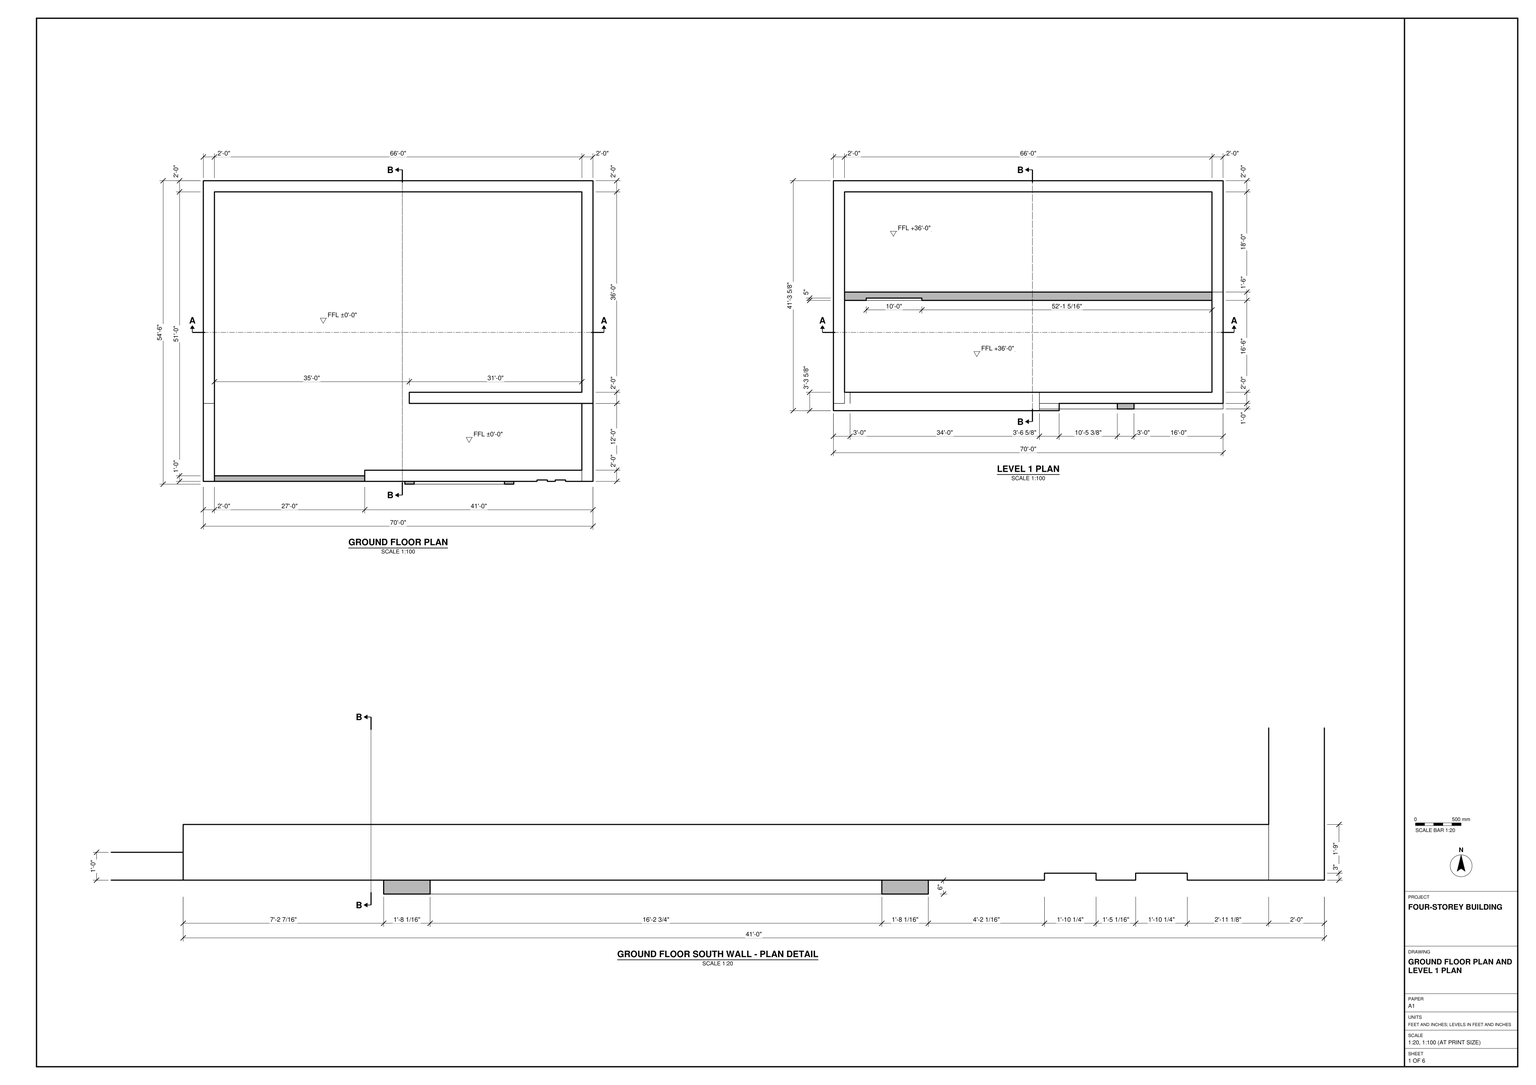
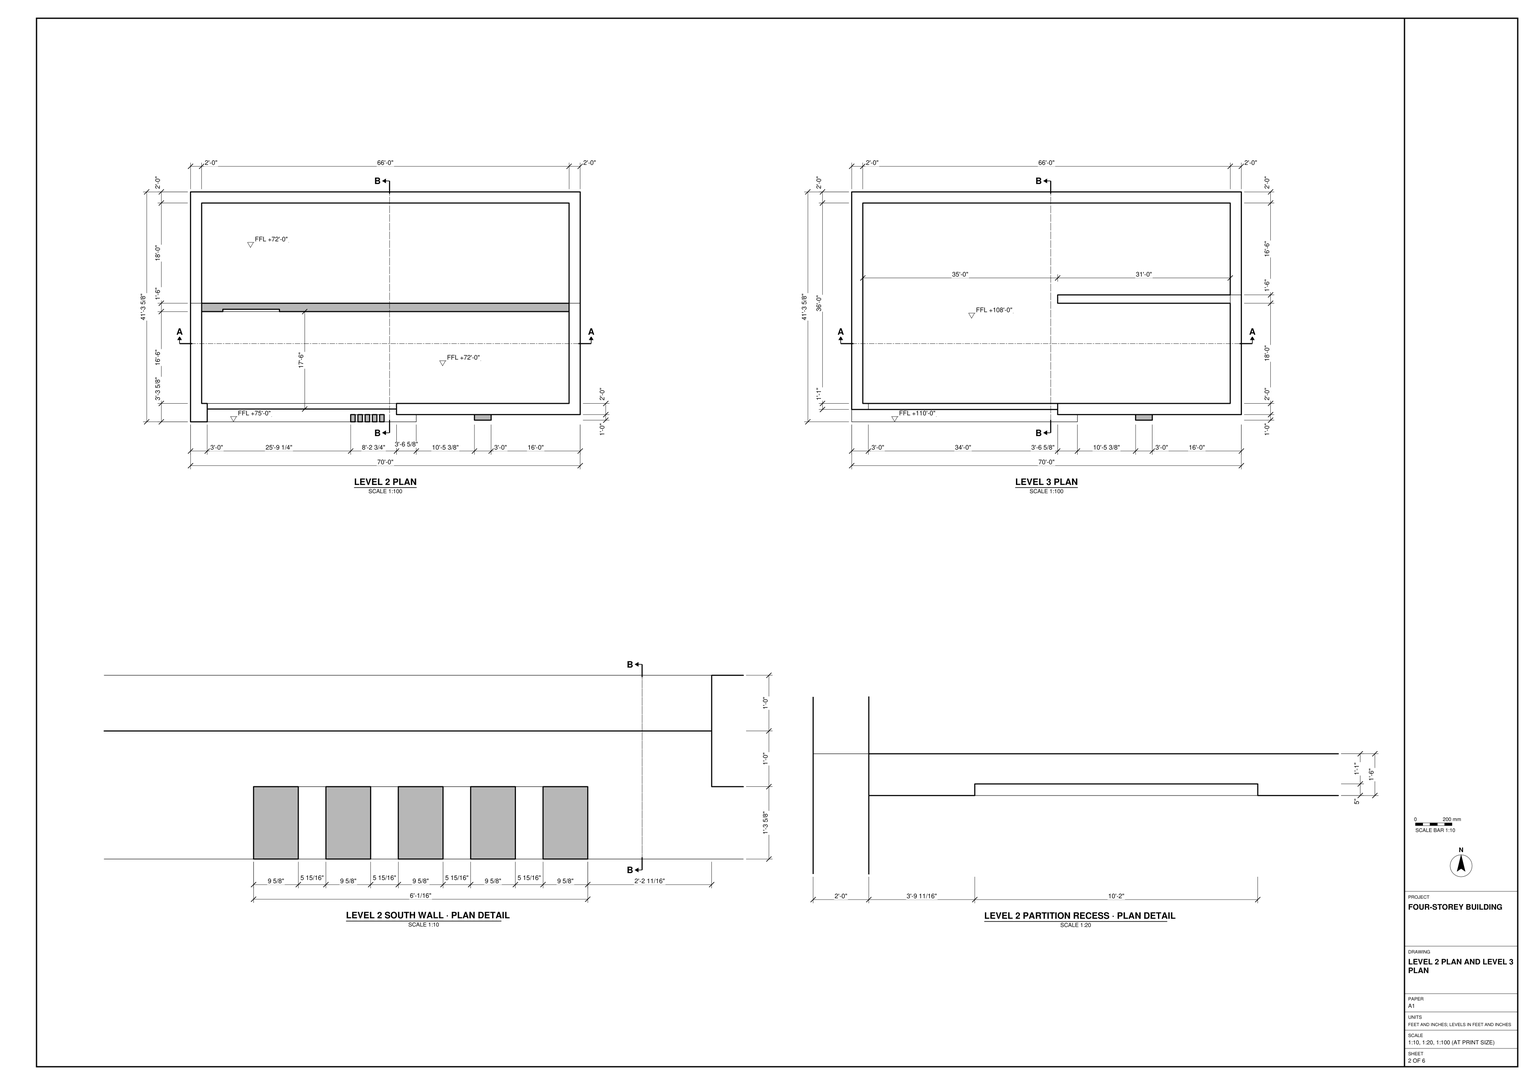
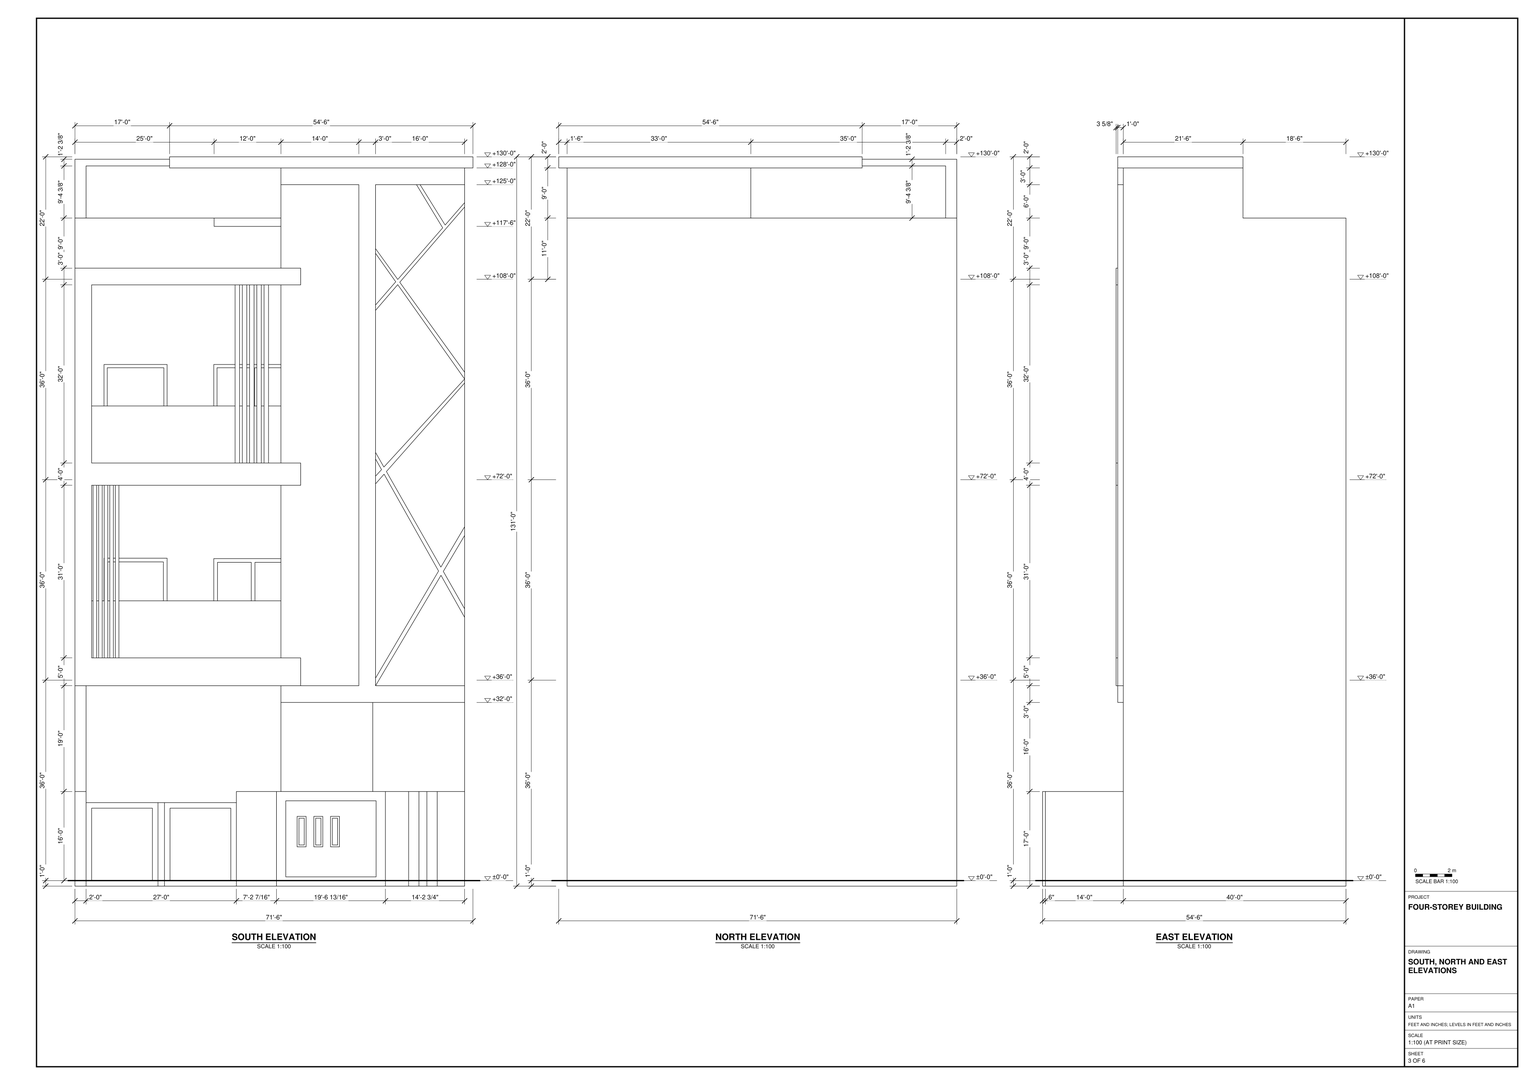
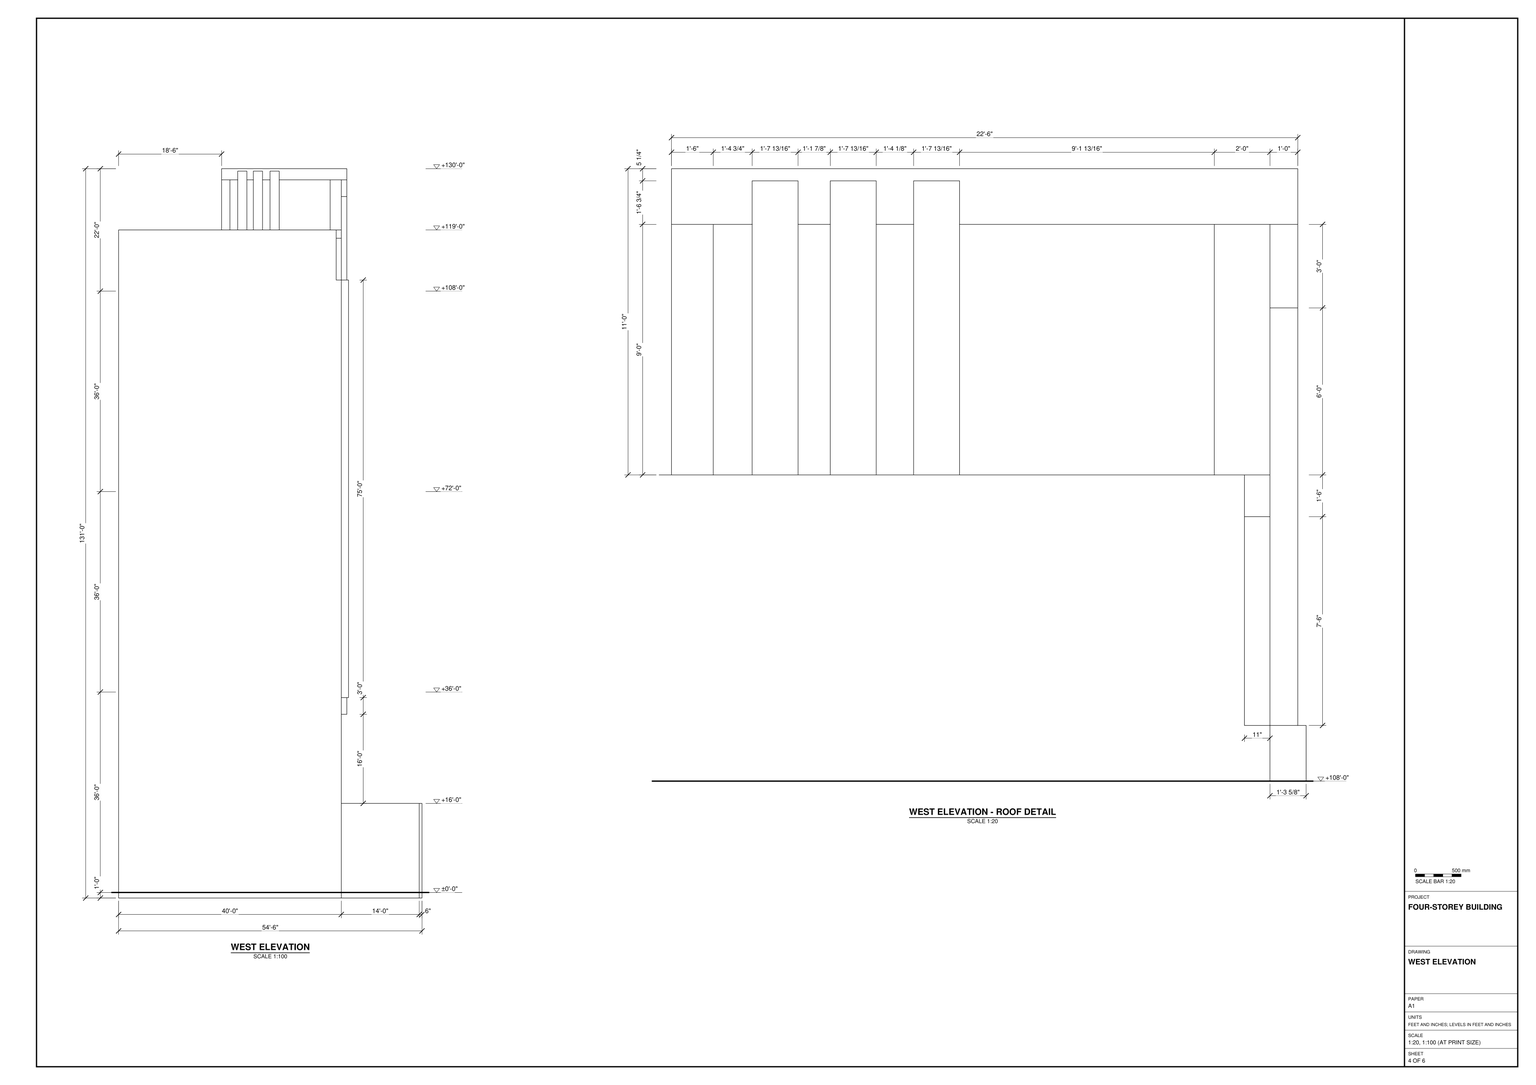
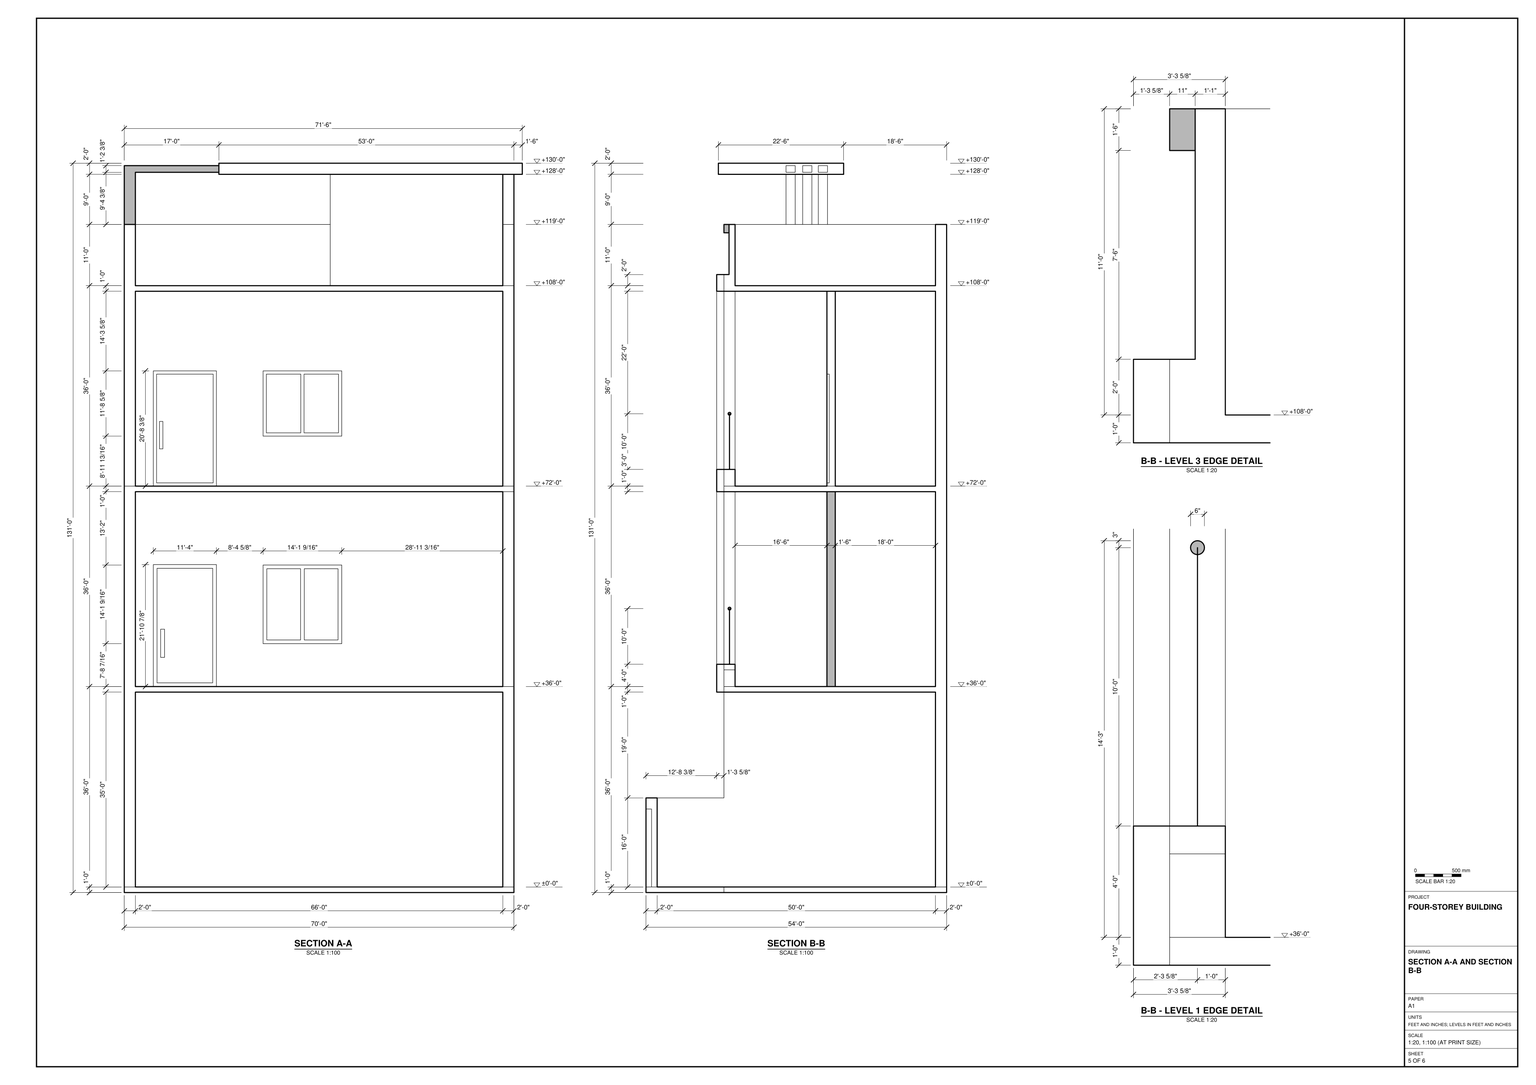
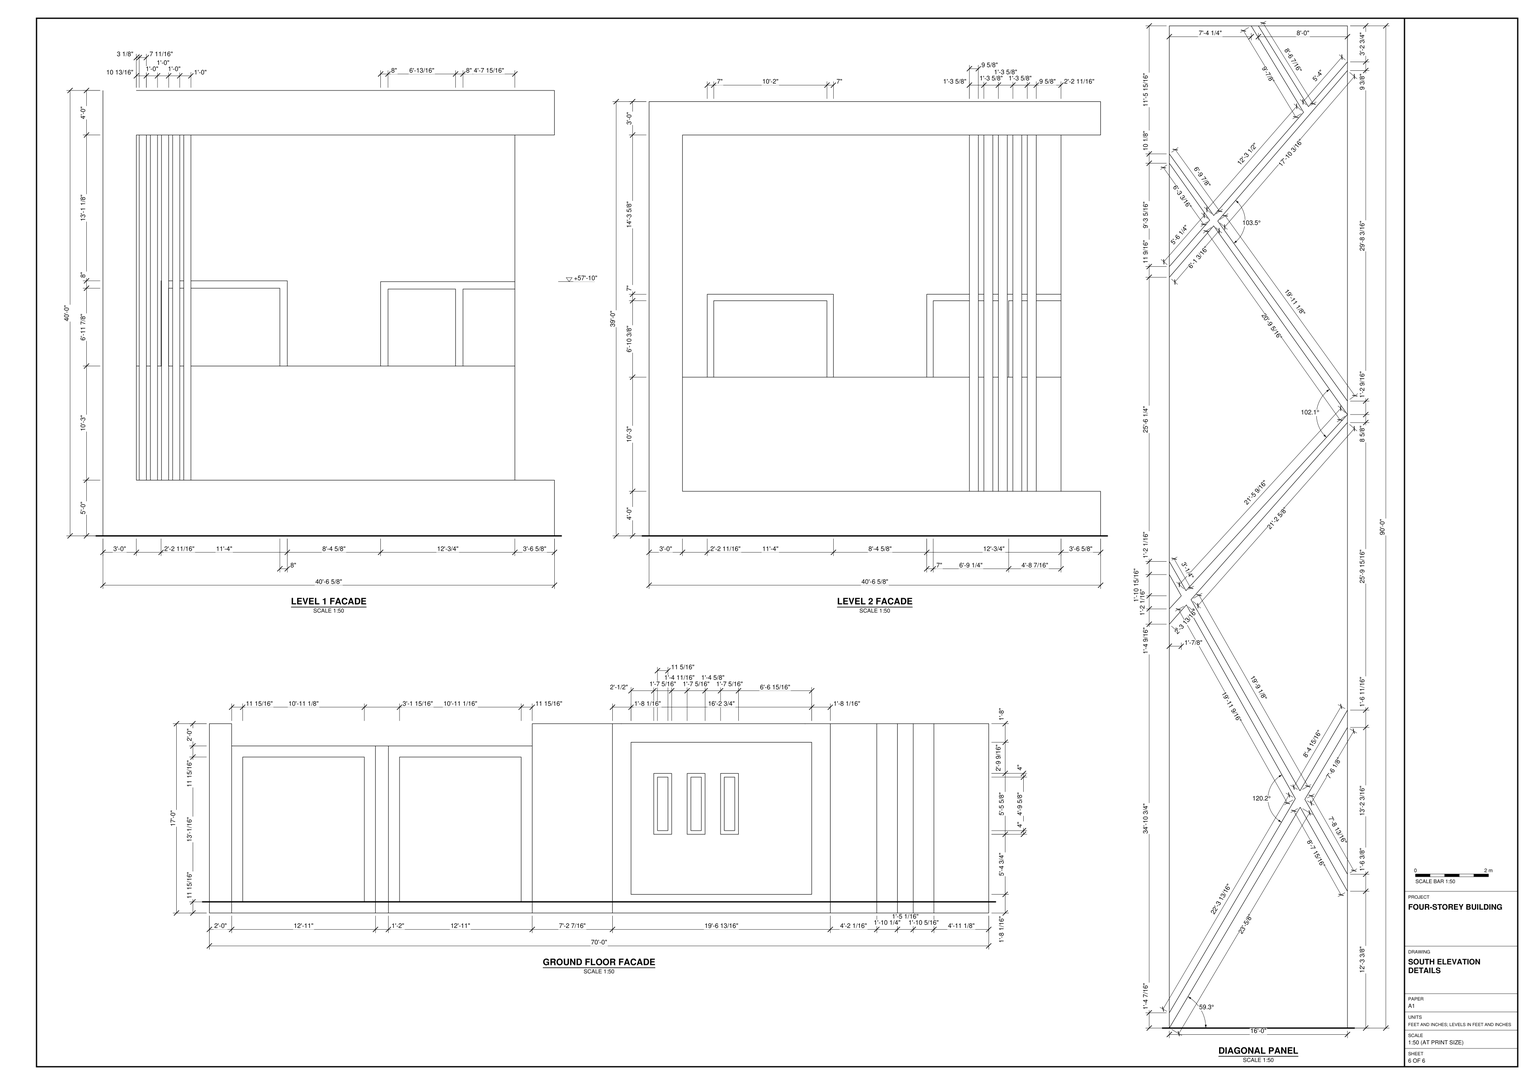
Build the four-storey building in SketchUp from task_files/diagram_01.pdf. Work in feet and inches. The overall model extents, including projections, are 71'-6" east to west, 54'-6" north to south and 131'-0" from bottom to top. Set the floor levels at ±0'-0", +36'-0", +72'-0" and +108'-0".

Use the floor plans to lay out the perimeter walls, internal partitions and slabs at their drawn thicknesses. Extend the low ground-floor frontage south of the upper-storey walls. Follow the plan details for the partition recesses and the changes in depth along the south face. On that face, model the ground-floor openings and inset panel, then form the stacked recessed bays above. Place the projecting horizontal bands and vertical fins as shown, noting that the fins change position between bays. Model the tall panel with crossing diagonal strips to the east of the bays. Use the elevations to shape the stepped roofline and its cap.

Keep walls, slabs and roof elements in separate groups or components, and keep each furniture or joinery piece shown separate. Use components for repeated parts such as the fins. Any decor or loose items shown may be represented by suitable library components. Save one SketchUp model as output_files/four_storey_building_with_its_screened_south_elevation.skp.

# SketchUp Ruby script. Lengths in inches.
U = 1.inch
M = Sketchup.active_model
def pt(a) = Geom::Point3d.new(a.map { |v| v * U })
def face(e, loops, mat)
  f = e.add_face(loops[0].map { |a| pt(a) })
  loops[1..].each { |l| e.add_face(l.map { |a| pt(a) }).erase! }
  f.material = f.back_material = mat if mat
  f
end
# faces: each face lists its corners as indices into pts; further lists are holes
def faces(e, pts, list, mat = nil) = list.each { |f| face(e, (f[0].is_a?(Array) ? f : [f]).map { |l| l.map { |i| pts[i] } }, mat) }
# xy, xz, yz: faces in a plane at the given z, y or x. An outline is a flat list of corners, or four numbers for a rectangle; further outlines are holes
def ring(l) = l.size == 4 ? [[l[0], l[1]], [l[2], l[1]], [l[2], l[3]], [l[0], l[3]]] : l.each_slice(2).to_a
def flat(e, list, mat, &to3) = list.each { |f| face(e, (f[0].is_a?(Array) ? f : [f]).map { |l| ring(l).map { |u, v| to3.(u, v) } }, mat) }
def xy(e, z, list, mat = nil) = flat(e, list, mat) { |x, y| [x, y, z] }
def xz(e, y, list, mat = nil) = flat(e, list, mat) { |x, z| [x, y, z] }
def yz(e, x, list, mat = nil) = flat(e, list, mat) { |y, z| [x, y, z] }
def lines(e, pts, list) = list.each { |a, b| e.add_line(pt(pts[a]), pt(pts[b])) }
# prism: a flat outline (further loops are holes) pulled along v
def prism(e, loops, v, mat = nil)
  f = face(e, loops, mat); d = Geom::Vector3d.new(v.map { |x| x * U })
  f.pushpull(f.normal.samedirection?(d) ? d.length : -d.length)
end
def box(e, o, s, mat = nil) = prism(e, [[o, [o[0] + s[0], o[1], o[2]], [o[0] + s[0], o[1] + s[1], o[2]], [o[0], o[1] + s[1], o[2]]]], [0, 0, s[2]], mat)
def at(x, y, z, deg = 0) = Geom::Transformation.translation(pt([x, y, z])) * Geom::Transformation.rotation(ORIGIN, Z_AXIS, deg.degrees)
def axes(o, x, y, z) = Geom::Transformation.new([*x, 0, *y, 0, *z, 0, *pt(o).to_a, 1])
def part(name) = M.definitions.add(name)
# library, detail: a bought-in or finely detailed component or shape, given as its bounding box
def library(name, o, s) = part(name).tap { |d| box(d.entities, o, s) }
def detail(e, o, s) = box(e.add_group.entities, o, s)
def put(e, d, t, mat = nil) = e.add_instance(d, t).tap { |i| i.material = mat if mat }
def group(e, t, mat = nil) = e.add_group.tap { |g| g.transformation = t; g.material = mat if mat }.entities
root = M.entities
M.materials.add("[0012_Bisque]").color = [214, 191, 164]
M.materials.add("[0012_Bisque]1").color = [255, 228, 196]
M.materials.add("[0021_DarkRed]").color = [94, 0, 0]
M.materials.add("[0021_DarkRed]1").color = [107, 0, 0]
M.materials.add("[0022_Maroon]").color = [63, 0, 0]
M.materials.add("[0027_PeachPuff]").color = [226, 194, 164]
M.materials.add("[0030_OldLace]").color = [237, 229, 215]
M.materials.add("[0042_Sienna]").color = [117, 60, 32]
M.materials.add("[0048_PaleGoldenrod]").color = [238, 232, 170]
M.materials.add("[0136_Charcoal]").color = [35, 35, 35]
M.materials.add("[Cladding Siding Tan]").color = [204, 97, 36]
M.materials.add("[Cladding Stucco White]").color = [200, 200, 200]
M.materials.add("[Granite Brown]").color = [126, 104, 91]
M.materials.add("[Granite Dark Gray]").color = [69, 68, 68]
M.materials.add("[Modern Siding]").color = [191, 132, 100]
M.materials.add("[Stone Flagstone Ashlar]").color = [175, 116, 102]
M.materials.add("[Stone Masonry Multi]").color = [182, 175, 164]
M.materials.add("[Translucent Glass Gray]").color = [198, 198, 198]
M.materials["[Translucent Glass Gray]"].alpha = 0.5
M.materials.add("[Translucent Glass Gray]1").color = [128, 128, 128]
M.materials["[Translucent Glass Gray]1"].alpha = 0.5
M.materials.add("[Wood Bamboo]").color = [177, 105, 43]
M.materials.add("[Wood Cherry Original]").color = [152, 86, 42]
xy(root,0,[[0,6,24,174],[24,6,24,174,840,174,840,6,780.9,6,780.9,9,758.64,9,758.64,6,741.58,6,741.58,9,719.33,9,719.33,6],[0,174,840,654]])
xy(root,0,[[434.43,0,669.25,6]],"[0012_Bisque]1")
xy(root,12,[[24,18,348,18,348,30,816,30,816,174,444,174,444,198,816,198,816,630,24,630]],"[Granite Dark Gray]")
xy(root,20.04,[[454.47,0,649.21,6]],"[0012_Bisque]1")
xy(root,84.76,[[478.96,0,498.27,6],[514.96,0,534.27,6],[550.96,0,570.27,6]])
xy(root,88.76,[[482.96,0,494.27,6],[518.96,0,530.27,6],[554.96,0,566.27,6]])
xy(root,146.39,[[482.96,0,494.27,6],[518.96,0,530.27,6],[554.96,0,566.27,6]])
xy(root,150.39,[[478.96,0,498.27,6],[514.96,0,534.27,6],[550.96,0,570.27,6]])
xy(root,180,[[24,6,348,18]])
xy(root,183.96,[[454.47,0,649.21,6]],"[0012_Bisque]1")
xy(root,204,[[0,6,24,174]],"[0012_Bisque]")
xy(root,204,[[434.43,0,669.25,6],[348,6,719.33,6,719.33,9,741.58,9,741.58,6,758.64,6,758.64,9,780.9,9,780.9,6,840,6,840,174,816,174,816,30,348,30]],"[0012_Bisque]1")
xy(root,396,[[444,162,840,174]],"[0012_Bisque]1")
xy(root,432,[[444,158.4,486.63,162],[444,162,486.63,174]])
xy(root,432,[[486.63,162,612,174],[648,162,840,174]],"[0012_Bisque]1")
xy(root,432,[[0,158.4,0,174,24,174,24,630,816,630,816,198,444,198,444,158.4]],"[Wood Cherry Original]")
xy(root,444,[[24,396,816,414],[24,414,816,630]])
xy(root,444,[[24,198,816,396]],"[Granite Brown]")
xy(root,452,[[70.68,396,190.68,401]],"[0022_Maroon]")
xy(root,492,[[36,158.4,39.12,174],[39.12,158.4,46.81,174],[46.81,158.4,51.12,174],[51.12,158.4,58.81,174],[58.81,158.4,63.12,174],
  [63.12,158.4,70.81,174],[70.81,158.4,75.12,174],[75.12,158.4,82.81,174],[82.81,158.4,87.12,174],[87.12,158.4,94.81,174]])
xy(root,492,[[94.81,158.4,486.63,158.4,486.63,174,444,174,444,186,36,186,36,174,94.81,174]],"[0012_Bisque]")
xy(root,492,[[36,186,444,198]],"[0012_Bisque]1")
xy(root,698.875,[[70.68,396,190.68,401]],"[0022_Maroon]")
xy(root,864,[[86.35,193.11,83.24,193.52,80.35,194.72,77.86,196.63,75.96,199.11,74.76,202.01,74.35,205.11,74.76,208.22,75.96,211.11,77.86,213.6,80.35,215.51,83.24,216.71,86.35,217.11,89.45,216.71,92.35,215.51,94.83,213.6,96.74,211.11,97.9375,208.22,98.35,205.11,97.9375,202.01,96.74,199.11,94.83,196.63,92.35,194.72,89.45,193.52],[170.35,193.11,167.24,193.52,164.35,194.72,161.86,196.63,159.96,199.11,158.76,202.01,158.35,205.11,158.76,208.22,159.96,211.11,161.86,213.6,164.35,215.51,167.24,216.71,170.35,217.11,173.45,216.71,176.35,215.51,178.83,213.6,180.74,211.11,181.9375,208.22,182.35,205.11,181.9375,202.01,180.74,199.11,178.83,196.63,176.35,194.72,173.45,193.52],[254.35,193.11,251.24,193.52,248.35,194.72,245.86,196.63,243.96,199.11,242.76,202.01,242.35,205.11,242.76,208.22,243.96,211.11,245.86,213.6,248.35,215.51,251.24,216.71,254.35,217.11,257.45,216.71,260.35,215.51,262.83,213.6,264.74,211.11,265.9375,208.22,266.35,205.11,265.9375,202.01,264.74,199.11,262.83,196.63,260.35,194.72,257.45,193.52],[338.35,193.11,335.24,193.52,332.35,194.72,329.86,196.63,327.96,199.11,326.76,202.01,326.35,205.11,326.76,208.22,327.96,211.11,329.86,213.6,332.35,215.51,335.24,216.71,338.35,217.11,341.45,216.71,344.35,215.51,346.83,213.6,348.74,211.11,349.9375,208.22,350.35,205.11,349.9375,202.01,348.74,199.11,346.83,196.63,344.35,194.72,341.45,193.52],[24,396,816,414],
  [24,414,816,630]])
xy(root,864,[[[36,158.4,36,198,24,198,24,396,816,396,816,198,444,198,444,174,486.63,174,486.63,158.4,94.81,158.4,94.81,174,87.12,174,87.12,158.4,82.81,158.4,82.81,174,75.12,174,75.12,158.4,70.81,158.4,70.81,174,63.12,174,63.12,158.4,58.81,158.4,58.81,174,51.12,174,51.12,158.4,46.81,158.4,46.81,174,39.12,174,39.12,158.4],[170.35,193.11,173.45,193.52,176.35,194.72,178.83,196.63,180.74,199.11,181.9375,202.01,182.35,205.11,181.9375,208.22,180.74,211.11,178.83,213.6,176.35,215.51,173.45,216.71,170.35,217.11,167.24,216.71,164.35,215.51,161.86,213.6,159.96,211.11,158.76,208.22,158.35,205.11,158.76,202.01,159.96,199.11,161.86,196.63,164.35,194.72,167.24,193.52],[254.35,193.11,257.45,193.52,260.35,194.72,262.83,196.63,264.74,199.11,265.9375,202.01,266.35,205.11,265.9375,208.22,264.74,211.11,262.83,213.6,260.35,215.51,257.45,216.71,254.35,217.11,251.24,216.71,248.35,215.51,245.86,213.6,243.96,211.11,242.76,208.22,242.35,205.11,242.76,202.01,243.96,199.11,245.86,196.63,248.35,194.72,251.24,193.52],[338.35,193.11,341.45,193.52,344.35,194.72,346.83,196.63,348.74,199.11,349.9375,202.01,350.35,205.11,349.9375,208.22,348.74,211.11,346.83,213.6,344.35,215.51,341.45,216.71,338.35,217.11,335.24,216.71,332.35,215.51,329.86,213.6,327.96,211.11,326.76,208.22,326.35,205.11,326.76,202.01,327.96,199.11,329.86,196.63,332.35,194.72,335.24,193.52],[86.35,193.11,89.45,193.52,92.35,194.72,94.83,196.63,96.74,199.11,97.9375,202.01,98.35,205.11,97.9375,208.22,96.74,211.11,94.83,213.6,92.35,215.51,89.45,216.71,86.35,217.11,83.24,216.71,80.35,215.51,77.86,213.6,75.96,211.11,74.76,208.22,74.35,205.11,74.76,202.01,75.96,199.11,77.86,196.63,80.35,194.72,83.24,193.52]]],"[Wood Cherry Original]")
xy(root,876,[[24,414,816,630]])
xy(root,876,[[24,198,816,396]],"[Granite Brown]")
xy(root,883,[[69.68,396,191.68,401]],"[0022_Maroon]")
xy(root,912,[[345.25,158.4,354.89,174],[360.85,158.4,370.49,174],[376.45,158.4,386.09,174],[392.05,158.4,401.6875,174],[407.65,158.4,417.29,174]])
xy(root,912,[[36,158.4,345.25,158.4,345.25,174,417.29,174,417.29,158.4,486.63,158.4,486.63,174,444,174,444,186,36,186],[354.89,158.4,360.85,174],[370.49,158.4,376.45,174],[386.09,158.4,392.05,174],[401.6875,158.4,407.65,174]],"[0012_Bisque]")
xy(root,912,[[36,186,444,198]],"[0012_Bisque]1")
xy(root,1117.39,[[69.68,396,191.68,401]],"[0022_Maroon]")
xy(root,1296,[[78.92,203.6875,75.8125,204.1,72.92,205.3,70.43,207.2,68.53,209.6875,67.33,212.58,66.92,215.6875,67.33,218.79,68.53,221.6875,70.43,224.17,72.92,226.08,75.8125,227.28,78.92,227.6875,82.02,227.28,84.92,226.08,87.4,224.17,89.3125,221.6875,90.51,218.79,90.92,215.6875,90.51,212.58,89.3125,209.6875,87.4,207.2,84.92,205.3,82.02,204.1],[162.92,203.6875,159.8125,204.1,156.92,205.3,154.43,207.2,152.53,209.6875,151.33,212.58,150.92,215.6875,151.33,218.79,152.53,221.6875,154.43,224.17,156.92,226.08,159.8125,227.28,162.92,227.6875,166.02,227.28,168.92,226.08,171.4,224.17,173.3125,221.6875,174.51,218.79,174.92,215.6875,174.51,212.58,173.3125,209.6875,171.4,207.2,168.92,205.3,166.02,204.1],[246.92,203.6875,243.8125,204.1,240.92,205.3,238.43,207.2,236.53,209.6875,235.33,212.58,234.92,215.6875,235.33,218.79,236.53,221.6875,238.43,224.17,240.92,226.08,243.8125,227.28,246.92,227.6875,250.02,227.28,252.92,226.08,255.4,224.17,257.3125,221.6875,258.51,218.79,258.92,215.6875,258.51,212.58,257.3125,209.6875,255.4,207.2,252.92,205.3,250.02,204.1],[330.92,203.6875,327.8125,204.1,324.92,205.3,322.43,207.2,320.53,209.6875,319.33,212.58,318.92,215.6875,319.33,218.79,320.53,221.6875,322.43,224.17,324.92,226.08,327.8125,227.28,330.92,227.6875,334.02,227.28,336.92,226.08,339.4,224.17,341.3125,221.6875,342.51,218.79,342.92,215.6875,342.51,212.58,341.3125,209.6875,339.4,207.2,336.92,205.3,334.02,204.1],[24,396,816,414],
  [24,396,816,630]])
xy(root,1296,[[[36,158.4,36,198,24,198,24,396,816,396,816,198,444,198,444,174,486.63,174,486.63,158.4,417.29,158.4,417.29,174,407.65,174,407.65,158.4,401.6875,158.4,401.6875,174,392.05,174,392.05,158.4,386.09,158.4,386.09,174,376.45,174,376.45,158.4,370.49,158.4,370.49,174,360.85,174,360.85,158.4,354.89,158.4,354.89,174,345.25,174,345.25,158.4],[162.92,203.6875,166.02,204.1,168.92,205.3,171.4,207.2,173.3125,209.6875,174.51,212.58,174.92,215.6875,174.51,218.79,173.3125,221.6875,171.4,224.17,168.92,226.08,166.02,227.28,162.92,227.6875,159.8125,227.28,156.92,226.08,154.43,224.17,152.53,221.6875,151.33,218.79,150.92,215.6875,151.33,212.58,152.53,209.6875,154.43,207.2,156.92,205.3,159.8125,204.1],[246.92,203.6875,250.02,204.1,252.92,205.3,255.4,207.2,257.3125,209.6875,258.51,212.58,258.92,215.6875,258.51,218.79,257.3125,221.6875,255.4,224.17,252.92,226.08,250.02,227.28,246.92,227.6875,243.8125,227.28,240.92,226.08,238.43,224.17,236.53,221.6875,235.33,218.79,234.92,215.6875,235.33,212.58,236.53,209.6875,238.43,207.2,240.92,205.3,243.8125,204.1],[330.92,203.6875,334.02,204.1,336.92,205.3,339.4,207.2,341.3125,209.6875,342.51,212.58,342.92,215.6875,342.51,218.79,341.3125,221.6875,339.4,224.17,336.92,226.08,334.02,227.28,330.92,227.6875,327.8125,227.28,324.92,226.08,322.43,224.17,320.53,221.6875,319.33,218.79,318.92,215.6875,319.33,212.58,320.53,209.6875,322.43,207.2,324.92,205.3,327.8125,204.1],[78.92,203.6875,82.02,204.1,84.92,205.3,87.4,207.2,89.3125,209.6875,90.51,212.58,90.92,215.6875,90.51,218.79,89.3125,221.6875,87.4,224.17,84.92,226.08,82.02,227.28,78.92,227.6875,75.8125,227.28,72.92,226.08,70.43,224.17,68.53,221.6875,67.33,218.79,66.92,215.6875,67.33,212.58,68.53,209.6875,70.43,207.2,72.92,205.3,75.8125,204.1]]],"[Wood Cherry Original]")
xy(root,1308,[[24,198,816,198,816,414,444,414,444,432,816,432,816,630,24,630]],"[0030_OldLace]")
xy(root,1332,[[0,158.4,486.63,158.4,486.63,174,444,174,444,185,0,185]],"[0012_Bisque]")
xy(root,1422,[[300,174,444,185]],"[0136_Charcoal]")
xy(root,1440,[[0,307.8,24,327.62],[0,343.74,24,363.55],[0,377.43,24,397.24]])
xy(root,1440,[[0,185,444,185,444,198,24,198,24,307.8,0,307.8],[0,327.62,24,343.74],[0,363.55,24,377.43],[0,397.24,24,397.24,24,630,816,630,816,432,840,432,840,654,0,654]],"[0030_OldLace]")
xy(root,1440,[[300,174,444,185]],"[0136_Charcoal]")
xy(root,1512,[[444,162,612,174],[648,162,840,174]],"[0027_PeachPuff]")
xy(root,1548,[[444,162,840,174],[444,174,444,198,816,198,816,414,444,414,444,432,840,432,840,174],[221.58,205.35,219.54,205.79,217.68,206.74,216.14,208.14,215,209.89,214.36,211.88,214.26,213.97,214.7,216.01,215.65,217.87,217.05,219.42,218.81,220.55,220.79,221.19,222.88,221.29,224.92,220.85,226.78,219.9,228.33,218.5,229.46,216.75,230.1,214.76,230.21,212.67,229.77,210.63,228.8125,208.77,227.41,207.22,225.66,206.09,223.67,205.45],[221.58,265.35,219.54,265.79,217.68,266.74,216.14,268.14,215,269.89,214.36,271.88,214.26,273.97,214.7,276.01,215.65,277.87,217.05,279.42,218.81,280.55,220.79,281.19,222.88,281.29,224.92,280.85,226.78,279.9,228.33,278.5,229.46,276.75,230.1,274.76,230.21,272.67,229.77,270.63,228.8125,268.77,227.41,267.22,225.66,266.09,223.67,265.45],[221.58,325.35,219.54,325.79,217.68,326.74,216.14,328.14,215,329.89,214.36,331.88,214.26,333.97,214.7,336.01,215.65,337.87,217.05,339.42,218.81,340.55,220.79,341.19,222.88,341.29,224.92,340.85,226.78,339.9,228.33,338.5,229.46,336.75,230.1,334.76,230.21,332.67,229.77,330.63,228.8125,328.77,227.41,327.22,225.66,326.09,223.67,325.45],
  [221.58,385.35,219.54,385.79,217.68,386.74,216.14,388.14,215,389.89,214.36,391.88,214.26,393.97,214.7,396.01,215.65,397.87,217.05,399.42,218.81,400.55,220.79,401.19,222.88,401.29,224.92,400.85,226.78,399.9,228.33,398.5,229.46,396.75,230.1,394.76,230.21,392.67,229.77,390.63,228.8125,388.77,227.41,387.22,225.66,386.09,223.67,385.45]])
xy(root,1548,[[[204,162,204,432,444,432,444,414,816,414,816,198,444,198,444,162],[221.58,325.35,223.67,325.45,225.66,326.09,227.41,327.22,228.8125,328.77,229.77,330.63,230.21,332.67,230.1,334.76,229.46,336.75,228.33,338.5,226.78,339.9,224.92,340.85,222.88,341.29,220.79,341.19,218.81,340.55,217.05,339.42,215.65,337.87,214.7,336.01,214.26,333.97,214.36,331.88,215,329.89,216.14,328.14,217.68,326.74,219.54,325.79],[221.58,385.35,223.67,385.45,225.66,386.09,227.41,387.22,228.8125,388.77,229.77,390.63,230.21,392.67,230.1,394.76,229.46,396.75,228.33,398.5,226.78,399.9,224.92,400.85,222.88,401.29,220.79,401.19,218.81,400.55,217.05,399.42,215.65,397.87,214.7,396.01,214.26,393.97,214.36,391.88,215,389.89,216.14,388.14,217.68,386.74,219.54,385.79],[221.58,205.35,223.67,205.45,225.66,206.09,227.41,207.22,228.8125,208.77,229.77,210.63,230.21,212.67,230.1,214.76,229.46,216.75,228.33,218.5,226.78,219.9,224.92,220.85,222.88,221.29,220.79,221.19,218.81,220.55,217.05,219.42,215.65,217.87,214.7,216.01,214.26,213.97,214.36,211.88,215,209.89,216.14,208.14,217.68,206.74,219.54,205.79],[221.58,265.35,223.67,265.45,225.66,266.09,227.41,267.22,228.8125,268.77,229.77,270.63,230.21,272.67,230.1,274.76,229.46,276.75,228.33,278.5,226.78,279.9,224.92,280.85,222.88,281.29,220.79,281.19,218.81,280.55,217.05,279.42,215.65,277.87,214.7,276.01,214.26,273.97,214.36,271.88,215,269.89,216.14,268.14,217.68,266.74,219.54,265.79]],[840,162,858,432]],"[Wood Bamboo]")
xy(root,1552.39,[[24,307.8,204,327.62],[24,343.74,204,363.55],[24,377.43,204,397.24]])
xy(root,1566.76,[[0,307.8,204,327.62],[0,343.74,204,363.55],[0,377.43,204,397.24]])
xy(root,1572,[[204,162,858,432]],"[Wood Bamboo]")
xz(root,0,[[[478.96,84.76,498.27,150.39],[482.96,88.76,494.27,146.39]],[[514.96,84.76,534.27,150.39],[518.96,88.76,530.27,146.39]],[[550.96,84.76,570.27,150.39],[554.96,88.76,566.27,146.39]]])
xz(root,0,[[[434.43,0,669.25,204],[454.47,20.04,649.21,183.96]]],"[0012_Bisque]1")
xz(root,6,[[[434.43,0,669.25,204],[454.47,20.04,649.21,183.96]],[[478.96,84.76,498.27,150.39],[482.96,88.76,494.27,146.39]],[[514.96,84.76,534.27,150.39],[518.96,88.76,530.27,146.39]],[[550.96,84.76,570.27,150.39],[554.96,88.76,566.27,146.39]],[482.96,88.76,494.27,146.39],
  [518.96,88.76,530.27,146.39],[554.96,88.76,566.27,146.39]])
xz(root,6,[[0,0,24,204],[669.25,0,719.33,204],[741.58,0,758.64,204],[780.9,0,840,204]],"[0012_Bisque]1")
xz(root,6,[[[24,0,179,180],[35.96,11.96,167.04,168.04]],[[193,0,348,180],[204.96,11.96,336.04,168.04]]],"[0021_DarkRed]1")
xz(root,6,[[[454.47,20.04,649.21,183.96],[478.96,84.76,498.27,150.39],[514.96,84.76,534.27,150.39],[550.96,84.76,570.27,150.39]]],"[0042_Sienna]")
xz(root,6,[[179,0,193,180]],"[Cladding Stucco White]")
xz(root,6,[[35.96,11.96,167.04,168.04],[204.96,11.96,336.04,168.04]],"[Modern Siding]")
xz(root,6,[[348,0,434.43,204]],"[Stone Flagstone Ashlar]")
xz(root,9,[[719.33,0,741.58,204],[758.64,0,780.9,204]],"[0042_Sienna]")
xz(root,18,[[24,12,348,180]],"[Modern Siding]")
xz(root,30,[[348,12,816,204]],"[0012_Bisque]1")
xz(root,158.4,[[0,432,486.63,432,486.63,492,36,492,36,864,486.63,864,486.63,912,36,912,36,1296,486.63,1296,486.63,1332,0,1332]],"[0012_Bisque]")
xz(root,158.4,[[39.12,492,46.81,864],[51.12,492,58.81,864],[63.12,492,70.81,864],[75.12,492,82.81,864],[87.12,492,94.81,864],
  [345.25,912,354.89,1296],[360.85,912,370.49,1296],[376.45,912,386.09,1296],[392.05,912,401.6875,1296],[407.65,912,417.29,1296]],"[0021_DarkRed]")
xz(root,162,[[444,396,840,396,840,432,648,432,648,1512,840,1512,840,1548,444,1548,444,1512,612,1512,612,432,444,432]],"[0027_PeachPuff]")
xz(root,162,[[204,1548,858,1572]],"[Wood Bamboo]")
xz(root,174,[[816,0,840,204],[444,396,444,432,612,432,612,1512,444,1512,444,1548,840,1548,840,1512,648,1512,648,432,840,432,840,396]])
xz(root,174,[[0,204,24,432]],"[0012_Bisque]")
xz(root,174,[[39.12,492,46.81,864],[51.12,492,58.81,864],[63.12,492,70.81,864],[75.12,492,82.81,864],[87.12,492,94.81,864],
  [345.25,912,354.89,1296],[360.85,912,370.49,1296],[376.45,912,386.09,1296],[392.05,912,401.6875,1296],[407.65,912,417.29,1296]],"[0021_DarkRed]")
xz(root,174,[[642,12,816,12,816,204,840,204,840,396,642,396]],"[0027_PeachPuff]")
xz(root,174,[[648,432,789.04,669.97,840,579.375,840,597.77,794.06,678.43,840,755.95,840,774.63,788.8,687.65,671.42,893.71,840,1084.54,840,1093.14,665.95,903.32,648,934.83,648,920.75,660.9,897.82,648,883.75,648,867.2,666.4,888.03,783.84,679.22,648,448.42],[840,1093.14,840,1107.69,700.2,1301.66,840,1463.89,840,1473.24,797.96,1424.95,744,1512,736.25,1512,792.71,1418.91,695.88,1307.65,648,1374.08,648,1363.97,691.5,1302.62,648,1252.64,648,1241.09,695.79,1296.55]],"[0048_PaleGoldenrod]")
xz(root,174,[[648,432,840,432,840,579.375,789.04,669.97],[648,448.42,783.84,679.22,666.4,888.03,648,867.2],[840,597.77,840,755.95,794.06,678.43],[788.8,687.65,840,774.63,840,1084.54,671.42,893.71],[648,883.75,660.9,897.82,648,920.75],
  [665.95,903.32,840,1093.14,695.79,1296.55,648,1241.09,648,934.83],[840,1107.69,840,1463.89,700.2,1301.66],[648,1252.64,691.5,1302.62,648,1363.97],[695.88,1307.65,792.71,1418.91,736.25,1512,648,1512,648,1374.08],[300,1422,444,1440],
  [797.96,1424.95,840,1473.24,840,1512,744,1512]],"[0136_Charcoal]")
xz(root,174,[[444,12,642,396],[486.63,432,612,432,612,1512,444,1512,444,1332,486.63,1332,486.63,1296,444,1296,444,912,486.63,912,486.63,864,444,864,444,492,486.63,492]],"[Cladding Siding Tan]")
xz(root,185,[[300,1422,444,1440]])
xz(root,185,[[0,1332,444,1332,444,1422,300,1422,300,1440,0,1440]],"[0027_PeachPuff]")
xz(root,186,[[36,609,444,612],[36,1029,444,1032]])
xz(root,186,[[36,492,444,609],[36,912,444,1029]],"[Translucent Glass Gray]1")
xz(root,198,[[24,444,36,864],[24,876,36,1296]])
xz(root,198,[[36,444,36,492,444,492,444,864,816,864,816,444]],"[0012_Bisque]1")
xz(root,198,[[444,12,816,432]],"[0027_PeachPuff]")
xz(root,198,[[24,1308,444,1440],[444,1308,816,1548]],"[0030_OldLace]")
xz(root,198,[[36,876,36,912,444,912,444,1296,816,1296,816,876]],"[Stone Masonry Multi]")
xz(root,307.8,[[0,1440,24,1440,24,1552.39,204,1552.39,204,1566.76,0,1566.76]])
xz(root,327.62,[[0,1440,0,1566.76,204,1566.76,204,1552.39,24,1552.39,24,1440]])
xz(root,343.74,[[0,1440,24,1440,24,1552.39,204,1552.39,204,1566.76,0,1566.76]])
xz(root,363.55,[[0,1440,0,1566.76,204,1566.76,204,1552.39,24,1552.39,24,1440]])
xz(root,377.43,[[0,1440,24,1440,24,1552.39,204,1552.39,204,1566.76,0,1566.76]])
xz(root,396,[[[62.68,444,198.68,706.875],[70.68,452,190.68,698.875]],[[299.28,536.41,468.84,705.97],[388.06,544.41,460.84,697.97],[307.28,544.41,380.06,697.97]],[[62.68,876,198.68,1124.39],[69.68,883,191.68,1117.39]],[[299.28,983.8,468.84,1124.39],[387.56,990.8,461.84,1117.39],[306.28,990.8,380.56,1117.39]]],"[0022_Maroon]")
xz(root,396,[[[24,444,62.68,444,62.68,706.875,198.68,706.875,198.68,444,816,444,816,864,24,864],[299.28,536.41,468.84,705.97]],[[24,876,62.68,876,62.68,1124.39,198.68,1124.39,198.68,876,816,876,816,1296,24,1296],[299.28,983.8,468.84,1124.39]]],"[Stone Masonry Multi]")
xz(root,396,[[307.28,544.41,380.06,697.97],[388.06,544.41,460.84,697.97],[306.28,990.8,380.56,1117.39],[387.56,990.8,461.84,1117.39]],"[Translucent Glass Gray]")
xz(root,397.24,[[0,1440,0,1566.76,204,1566.76,204,1552.39,24,1552.39,24,1440]])
xz(root,401,[[[70.68,452,190.68,698.875],[78.43,506.89,86.87,567.58]],[[69.68,883,191.68,1117.39],[75.96,956.3125,83.27,1015.4375]]],"[0022_Maroon]")
xz(root,401,[[78.43,506.89,86.87,567.58],[75.96,956.3125,83.27,1015.4375]],"[0030_OldLace]")
xz(root,414,[[24,444,816,864],[24,876,816,1296]])
xz(root,414,[[444,1308,816,1548]],"[0030_OldLace]")
xz(root,432,[[444,1308,444,1548,840,1548,840,1440,816,1440,816,1308]],"[0030_OldLace]")
xz(root,432,[[204,1548,858,1572]],"[Wood Bamboo]")
xz(root,630,[[24,444,816,864],[24,876,816,1296]])
xz(root,630,[[24,12,816,432]],"[0012_Bisque]")
xz(root,630,[[24,1308,816,1440]],"[0030_OldLace]")
xz(root,654,[[0,0,840,12]])
xz(root,654,[[0,12,840,1440]],"[0030_OldLace]")
yz(root,0,[[6,0,174,12],[174,0,654,12],[307.8,1440,327.62,1566.76],[343.74,1440,363.55,1566.76],[377.43,1440,397.24,1566.76]])
yz(root,0,[[158.4,432,174,1332]],"[0012_Bisque]")
yz(root,0,[[6,12,174,204]],"[0012_Bisque]1")
yz(root,0,[[174,12,174,1332,185,1332,185,1440,654,1440,654,12]],"[0030_OldLace]")
yz(root,24,[[6,0,174,12],[6,12,18,180],[396,444,414,864],[414,444,630,864],[396,876,414,1296],
  [414,876,630,1296],[307.8,1440,327.62,1552.39],[343.74,1440,363.55,1552.39],[377.43,1440,397.24,1552.39]])
yz(root,24,[[18,12,630,12,630,432,174,432,174,204,6,204,6,180,18,180]],"[0012_Bisque]")
yz(root,24,[[198,1308,630,1440]],"[0030_OldLace]")
yz(root,24,[[198,444,396,864],[198,876,396,1296]],"[Stone Masonry Multi]")
yz(root,36,[[[158.4,492,198,864],[186,609,185.22,609.1,184.5,609.4,183.88,609.88,183.4,610.5,183.1,611.22,183,612,183.1,612.78,183.4,613.5,183.88,614.12,184.5,614.6,185.22,614.9,186,615,186.78,614.9,187.5,614.6,188.12,614.12,188.6,613.5,188.9,612.78,189,612,188.9,611.22,188.6,610.5,188.12,609.88,187.5,609.4,186.78,609.1]]])
yz(root,36,[[[158.4,912,198,1296],[186,1029,185.22,1029.1,184.5,1029.4,183.88,1029.88,183.4,1030.5,183.1,1031.22,183,1032,183.1,1032.78,183.4,1033.5,183.88,1034.12,184.5,1034.6,185.22,1034.9,186,1035,186.78,1034.9,187.5,1034.6,188.12,1034.12,188.6,1033.5,188.9,1032.78,189,1032,188.9,1031.22,188.6,1030.5,188.12,1029.88,187.5,1029.4,186.78,1029.1]]],"[0012_Bisque]")
yz(root,39.12,[[158.4,492,174,864]],"[0021_DarkRed]")
yz(root,46.81,[[158.4,492,174,864]],"[0021_DarkRed]")
yz(root,51.12,[[158.4,492,174,864]],"[0021_DarkRed]")
yz(root,58.81,[[158.4,492,174,864]],"[0021_DarkRed]")
yz(root,63.12,[[158.4,492,174,864]],"[0021_DarkRed]")
yz(root,69.68,[[396,883,401,1117.39]],"[0022_Maroon]")
yz(root,70.68,[[396,452,401,698.875]],"[0022_Maroon]")
yz(root,70.81,[[158.4,492,174,864]],"[0021_DarkRed]")
yz(root,75.12,[[158.4,492,174,864]],"[0021_DarkRed]")
yz(root,82.81,[[158.4,492,174,864]],"[0021_DarkRed]")
yz(root,87.12,[[158.4,492,174,864]],"[0021_DarkRed]")
yz(root,94.81,[[158.4,492,174,864]],"[0021_DarkRed]")
yz(root,190.68,[[396,452,401,698.875]],"[0022_Maroon]")
yz(root,191.68,[[396,883,401,1117.39]],"[0022_Maroon]")
yz(root,204,[[307.8,1552.39,327.62,1566.76],[343.74,1552.39,363.55,1566.76],[377.43,1552.39,397.24,1566.76]])
yz(root,204,[[[162,1548,432,1572],[377.43,1552.39,397.24,1566.76],[343.74,1552.39,363.55,1566.76],[307.8,1552.39,327.62,1566.76]]],"[Wood Bamboo]")
yz(root,300,[[174,1422,185,1440]],"[0136_Charcoal]")
yz(root,345.25,[[158.4,912,174,1296]],"[0021_DarkRed]")
yz(root,348,[[6,12,18,180]])
yz(root,348,[[18,12,18,180,6,180,6,204,30,204,30,12]],"[0012_Bisque]1")
yz(root,354.89,[[158.4,912,174,1296]],"[0021_DarkRed]")
yz(root,360.85,[[158.4,912,174,1296]],"[0021_DarkRed]")
yz(root,370.49,[[158.4,912,174,1296]],"[0021_DarkRed]")
yz(root,376.45,[[158.4,912,174,1296]],"[0021_DarkRed]")
yz(root,386.09,[[158.4,912,174,1296]],"[0021_DarkRed]")
yz(root,392.05,[[158.4,912,174,1296]],"[0021_DarkRed]")
yz(root,401.6875,[[158.4,912,174,1296]],"[0021_DarkRed]")
yz(root,407.65,[[158.4,912,174,1296]],"[0021_DarkRed]")
yz(root,417.29,[[158.4,912,174,1296]],"[0021_DarkRed]")
yz(root,434.43,[[0,0,6,204]],"[0012_Bisque]1")
yz(root,444,[[186,609,185.22,609.1,184.5,609.4,183.88,609.88,183.4,610.5,183.1,611.22,183,612,183.1,612.78,183.4,613.5,183.88,614.12,184.5,614.6,185.22,614.9,186,615,186.78,614.9,187.5,614.6,188.12,614.12,188.6,613.5,188.9,612.78,189,612,188.9,611.22,188.6,610.5,188.12,609.88,187.5,609.4,186.78,609.1],[186,1029,185.22,1029.1,184.5,1029.4,183.88,1029.88,183.4,1030.5,183.1,1031.22,183,1032,183.1,1032.78,183.4,1033.5,183.88,1034.12,184.5,1034.6,185.22,1034.9,186,1035,186.78,1034.9,187.5,1034.6,188.12,1034.12,188.6,1033.5,188.9,1032.78,189,1032,188.9,1031.22,188.6,1030.5,188.12,1029.88,187.5,1029.4,186.78,1029.1],[174,1306,185,1308],[174,1308,185,1332],[185,1308,198,1440],
  [174,1422,185,1440]])
yz(root,444,[[174,12,198,432],[162,396,174,432],[[174,492,198,864],[186,609,186.78,609.1,187.5,609.4,188.12,609.88,188.6,610.5,188.9,611.22,189,612,188.9,612.78,188.6,613.5,188.12,614.12,187.5,614.6,186.78,614.9,186,615,185.22,614.9,184.5,614.6,183.88,614.12,183.4,613.5,183.1,612.78,183,612,183.1,611.22,183.4,610.5,183.88,609.88,184.5,609.4,185.22,609.1]],[[174,912,198,1296],[186,1029,186.78,1029.1,187.5,1029.4,188.12,1029.88,188.6,1030.5,188.9,1031.22,189,1032,188.9,1032.78,188.6,1033.5,188.12,1034.12,187.5,1034.6,186.78,1034.9,186,1035,185.22,1034.9,184.5,1034.6,183.88,1034.12,183.4,1033.5,183.1,1032.78,183,1032,183.1,1031.22,183.4,1030.5,183.88,1029.88,184.5,1029.4,185.22,1029.1]],[174,1332,185,1422],
  [174,1440,198,1548],[162,1512,174,1548]],"[0027_PeachPuff]")
yz(root,444,[[414,1308,432,1548]],"[0030_OldLace]")
yz(root,454.47,[[0,20.04,6,183.96]],"[0012_Bisque]1")
yz(root,478.96,[[0,84.76,6,150.39]])
yz(root,482.96,[[0,88.76,6,146.39]])
yz(root,486.63,[[158.4,864,174,912],[158.4,1296,174,1332]],"[0012_Bisque]")
yz(root,486.63,[[158.4,432,174,492]],"[0012_Bisque]1")
yz(root,494.27,[[0,88.76,6,146.39]])
yz(root,498.27,[[0,84.76,6,150.39]])
yz(root,514.96,[[0,84.76,6,150.39]])
yz(root,518.96,[[0,88.76,6,146.39]])
yz(root,530.27,[[0,88.76,6,146.39]])
yz(root,534.27,[[0,84.76,6,150.39]])
yz(root,550.96,[[0,84.76,6,150.39]])
yz(root,554.96,[[0,88.76,6,146.39]])
yz(root,566.27,[[0,88.76,6,146.39]])
yz(root,570.27,[[0,84.76,6,150.39]])
yz(root,612,[[162,432,174,1512]],"[0027_PeachPuff]")
yz(root,648,[[162,432,174,1512]],"[0027_PeachPuff]")
yz(root,649.21,[[0,20.04,6,183.96]],"[0012_Bisque]1")
yz(root,669.25,[[0,0,6,204]],"[0012_Bisque]1")
yz(root,719.33,[[6,0,9,204]],"[0042_Sienna]")
yz(root,741.58,[[6,0,9,204]],"[0042_Sienna]")
yz(root,758.64,[[6,0,9,204]],"[0042_Sienna]")
yz(root,780.9,[[6,0,9,204]],"[0042_Sienna]")
yz(root,816,[[396,444,414,864],[414,444,630,864],[396,876,414,1296],[414,876,630,1296]])
yz(root,816,[[30,12,174,204]],"[0012_Bisque]1")
yz(root,816,[[198,12,630,432]],"[0027_PeachPuff]")
yz(root,816,[[198,1308,414,1548],[432,1308,630,1440]],"[0030_OldLace]")
yz(root,816,[[198,444,396,864],[198,876,396,1296]],"[Stone Masonry Multi]")
yz(root,840,[[162,396,174,432]])
yz(root,840,[[6,0,174,204]],"[0012_Bisque]1")
yz(root,840,[[162,1512,174,1548]],"[0027_PeachPuff]")
yz(root,840,[[174,0,654,0,654,1440,432,1440,432,1548,174,1548]],"[0030_OldLace]")
yz(root,858,[[162,1548,432,1572]],"[Wood Bamboo]")
p = [[36,185.22,609.1],[36,186,609],[444,186,609],[444,185.22,609.1],[36,186.78,609.1],[444,186.78,609.1],
  [36,184.5,609.4],[444,184.5,609.4],[36,187.5,609.4],[444,187.5,609.4],[36,183.88,609.88],[444,183.88,609.88],
  [36,188.12,609.88],[444,188.12,609.88],[36,183.4,610.5],[444,183.4,610.5],[36,188.6,610.5],[444,188.6,610.5],
  [36,183.1,611.22],[444,183.1,611.22],[36,188.9,611.22],[444,188.9,611.22],[36,183,612],[444,183,612],
  [36,189,612],[444,189,612],[36,183.1,612.78],[444,183.1,612.78],[36,188.9,612.78],[444,188.9,612.78],
  [36,183.4,613.5],[444,183.4,613.5],[36,188.6,613.5],[444,188.6,613.5],[36,183.88,614.12],[444,183.88,614.12],
  [36,188.12,614.12],[444,188.12,614.12],[36,184.5,614.6],[444,184.5,614.6],[36,187.5,614.6],[444,187.5,614.6],
  [36,185.22,614.9],[444,185.22,614.9],[36,186.78,614.9],[444,186.78,614.9],[36,186,615],[444,186,615],
  [36,185.22,1029.1],[36,186,1029],[444,186,1029],[444,185.22,1029.1],[36,186.78,1029.1],[444,186.78,1029.1],
  [36,184.5,1029.4],[444,184.5,1029.4],[36,187.5,1029.4],[444,187.5,1029.4],[36,183.88,1029.88],[444,183.88,1029.88],
  [36,188.12,1029.88],[444,188.12,1029.88],[36,183.4,1030.5],[444,183.4,1030.5],[36,188.6,1030.5],[444,188.6,1030.5],
  [36,183.1,1031.22],[444,183.1,1031.22],[36,188.9,1031.22],[444,188.9,1031.22],[36,183,1032],[444,183,1032],
  [36,189,1032],[444,189,1032],[36,183.1,1032.78],[444,183.1,1032.78],[36,188.9,1032.78],[444,188.9,1032.78],
  [36,183.4,1033.5],[444,183.4,1033.5],[36,188.6,1033.5],[444,188.6,1033.5],[36,183.88,1034.12],[444,183.88,1034.12],
  [36,188.12,1034.12],[444,188.12,1034.12],[36,184.5,1034.6],[444,184.5,1034.6],[36,187.5,1034.6],[444,187.5,1034.6],
  [36,185.22,1034.9],[444,185.22,1034.9],[36,186.78,1034.9],[444,186.78,1034.9],[36,186,1035],[444,186,1035],
  [816,414,444],[840,414,444],[816,414,864],[840,414,864],[816,414,876],[840,414,876],
  [24,414,876],[0,414,876],[0,174,1296],[36,174,1296],[816,432,1308],[840,432,1308],
  [0,185,1306],[444,185,1306],[36,198,876],[36,174,876],[444,174,1296],[444,174,1306],
  [36,198,444],[36,174,444],[36,198,480],[36,174,480],[444,158.4,1306],[444,174,1308],
  [444,158.4,1308],[816,30,12],[816,6,12]]
faces(root,p,[[0,1,2,3],[1,4,5,2],[6,0,3,7],[4,8,9,5],[10,6,7,11],[8,12,13,9],[14,10,11,15],[12,16,17,13],
  [18,14,15,19],[16,20,21,17],[22,18,19,23],[20,24,25,21],[26,22,23,27],[24,28,29,25],[30,26,27,31],[28,32,33,29],
  [34,30,31,35],[32,36,37,33],[38,34,35,39],[36,40,41,37],[42,38,39,43],[40,44,45,41],[46,42,43,47],[44,46,47,45],
  [48,49,50,51],[49,52,53,50],[54,48,51,55],[52,56,57,53],[58,54,55,59],[56,60,61,57],[62,58,59,63],[60,64,65,61],
  [66,62,63,67],[64,68,69,65],[70,66,67,71],[68,72,73,69],[74,70,71,75],[72,76,77,73],[78,74,75,79],[76,80,81,77],
  [82,78,79,83],[80,84,85,81],[86,82,83,87],[84,88,89,85],[90,86,87,91],[88,92,93,89],[94,90,91,95],[92,94,95,93]],"[0136_Charcoal]")
lines(root,p,[[96,97],[98,99],[100,101],[102,103],[104,105],[106,107],[108,109],[110,111],[112,113],[114,115],[116,117],[113,118],
  [119,120],[121,122]])
